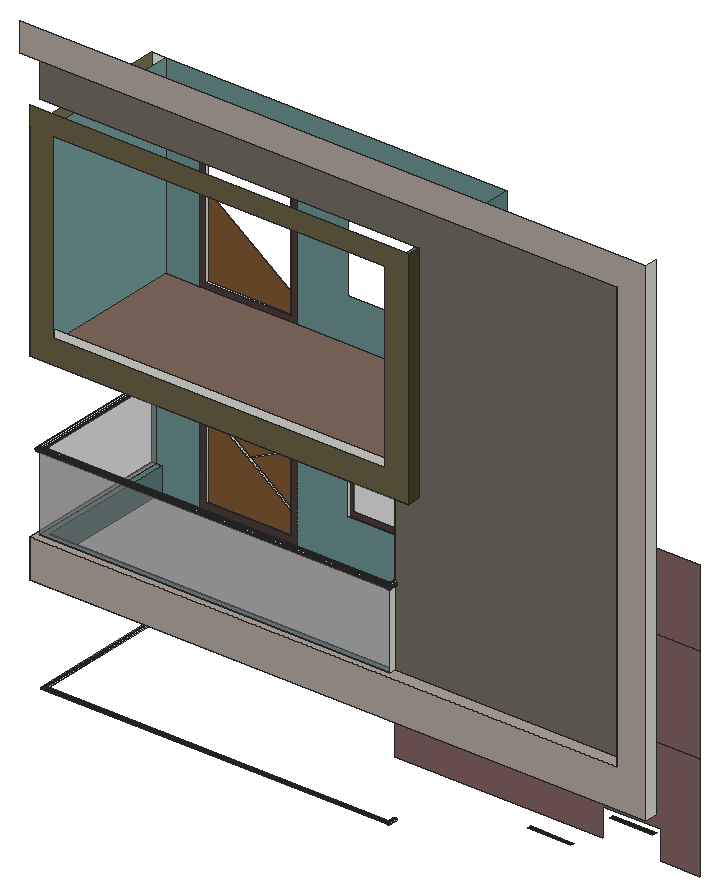
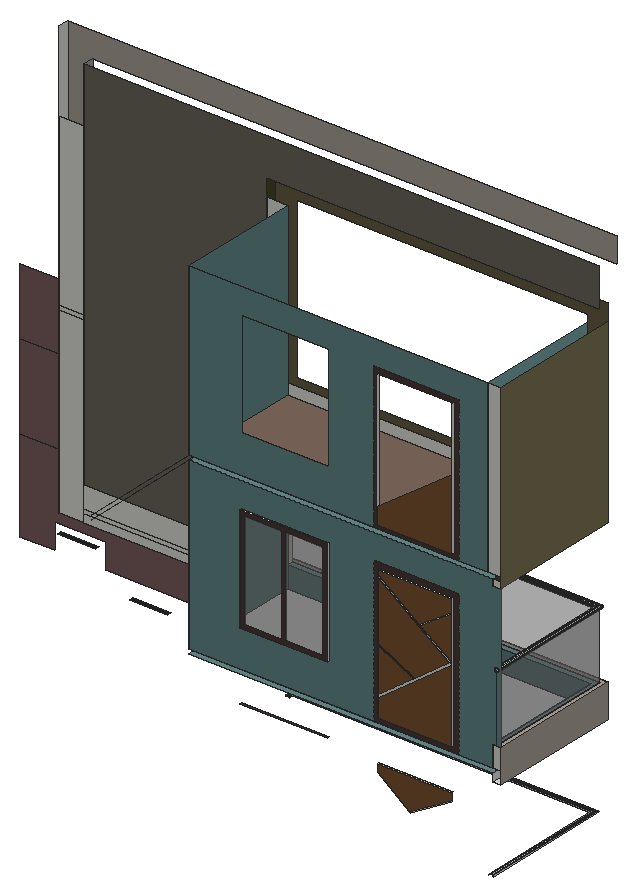
# SketchUp Ruby script. Lengths in inches.
U = 1.inch
M = Sketchup.active_model
def pt(a) = Geom::Point3d.new(a.map { |v| v * U })
def face(e, loops, mat)
  f = e.add_face(loops[0].map { |a| pt(a) })
  loops[1..].each { |l| e.add_face(l.map { |a| pt(a) }).erase! }
  f.material = f.back_material = mat if mat
  f
end
# faces: each face lists its corners as indices into pts; further lists are holes
def faces(e, pts, list, mat = nil) = list.each { |f| face(e, (f[0].is_a?(Array) ? f : [f]).map { |l| l.map { |i| pts[i] } }, mat) }
# xy, xz, yz: faces in a plane at the given z, y or x. An outline is a flat list of corners, or four numbers for a rectangle; further outlines are holes
def ring(l) = l.size == 4 ? [[l[0], l[1]], [l[2], l[1]], [l[2], l[3]], [l[0], l[3]]] : l.each_slice(2).to_a
def flat(e, list, mat, &to3) = list.each { |f| face(e, (f[0].is_a?(Array) ? f : [f]).map { |l| ring(l).map { |u, v| to3.(u, v) } }, mat) }
def xy(e, z, list, mat = nil) = flat(e, list, mat) { |x, y| [x, y, z] }
def xz(e, y, list, mat = nil) = flat(e, list, mat) { |x, z| [x, y, z] }
def yz(e, x, list, mat = nil) = flat(e, list, mat) { |y, z| [x, y, z] }
def lines(e, pts, list) = list.each { |a, b| e.add_line(pt(pts[a]), pt(pts[b])) }
# prism: a flat outline (further loops are holes) pulled along v
def prism(e, loops, v, mat = nil)
  f = face(e, loops, mat); d = Geom::Vector3d.new(v.map { |x| x * U })
  f.pushpull(f.normal.samedirection?(d) ? d.length : -d.length)
end
def box(e, o, s, mat = nil) = prism(e, [[o, [o[0] + s[0], o[1], o[2]], [o[0] + s[0], o[1] + s[1], o[2]], [o[0], o[1] + s[1], o[2]]]], [0, 0, s[2]], mat)
def at(x, y, z, deg = 0) = Geom::Transformation.translation(pt([x, y, z])) * Geom::Transformation.rotation(ORIGIN, Z_AXIS, deg.degrees)
def axes(o, x, y, z) = Geom::Transformation.new([*x, 0, *y, 0, *z, 0, *pt(o).to_a, 1])
def part(name) = M.definitions.add(name)
# library, detail: a bought-in or finely detailed component or shape, given as its bounding box
def library(name, o, s) = part(name).tap { |d| box(d.entities, o, s) }
def detail(e, o, s) = box(e.add_group.entities, o, s)
def put(e, d, t, mat = nil) = e.add_instance(d, t).tap { |i| i.material = mat if mat }
def group(e, t, mat = nil) = e.add_group.tap { |g| g.transformation = t; g.material = mat if mat }.entities
root = M.entities
M.materials.add("[0057_DarkKhaki]").color = [71, 69, 40]
M.materials.add("[0089_PaleTurquoise]").color = [103, 140, 140]
M.materials.add("[0089_PaleTurquoise]1").color = [120, 163, 163]
M.materials.add("[0089_PaleTurquoise]2").color = [93, 127, 127]
M.materials.add("[0119_RosyBrown]").color = [127, 96, 96]
M.materials.add("[0119_RosyBrown]1").color = [76, 58, 58]
M.materials.add("[0136_Charcoal]").color = [35, 35, 35]
M.materials.add("[Carrera Marble]").color = [193, 193, 193]
M.materials.add("[Cladding Stucco White]").color = [173, 163, 155]
M.materials.add("[Cladding Weathered]").color = [111, 105, 96]
M.materials.add("[Granite Brown]").color = [126, 104, 91]
M.materials.add("[Translucent Glass Gray]").color = [130, 130, 130]
M.materials["[Translucent Glass Gray]"].alpha = 0.5
M.materials.add("[Translucent Glass Gray]1").color = [128, 128, 128]
M.materials["[Translucent Glass Gray]1"].alpha = 0.5
M.materials.add("[Wood Floor]").color = [124, 84, 49]
M.materials.add("[Wood Lumber ButtJoined]").color = [102, 94, 69]
M.materials.add("[Wood Lumber ButtJoined]1").color = [127, 118, 87]
xy(root,1310.4375,[[1452,198,1560,208]],"[0136_Charcoal]")
xy(root,1388.4,[[375.6,546,584.4,551]])
xy(root,1404,[[726,546,973.25,552]],"[0119_RosyBrown]1")
xy(root,1406.375,[[1656,198,1764,208]],"[0136_Charcoal]")
xy(root,1452,[[240,167,240,546,264,546,264,198,1770,198,1770,167]])
xy(root,1476,[[353.9,283.84,350.8,284.25,347.9,285.44,345.42,287.35,343.51,289.84,342.31,292.73,341.9,295.84,342.31,298.94,343.51,301.84,345.42,304.32,347.9,306.23,350.8,307.43,353.9,307.84,357.01,307.43,359.9,306.23,362.39,304.32,364.29,301.84,365.49,298.94,365.9,295.84,365.49,292.73,364.29,289.84,362.39,287.35,359.9,285.44,357.01,284.25],[677.9,283.84,674.8,284.25,671.9,285.44,669.42,287.35,667.51,289.84,666.31,292.73,665.9,295.84,666.31,298.94,667.51,301.84,669.42,304.32,671.9,306.23,674.8,307.43,677.9,307.84,681.01,307.43,683.9,306.23,686.39,304.32,688.29,301.84,689.49,298.94,689.9,295.84,689.49,292.73,688.29,289.84,686.39,287.35,683.9,285.44,681.01,284.25],[1001.9,283.84,998.8,284.25,995.9,285.44,993.42,287.35,991.51,289.84,990.31,292.73,989.9,295.84,990.31,298.94,991.51,301.84,993.42,304.32,995.9,306.23,998.8,307.43,1001.9,307.84,1005.01,307.43,1007.9,306.23,1010.39,304.32,1012.29,301.84,1013.49,298.94,1013.9,295.84,1013.49,292.73,1012.29,289.84,1010.39,287.35,1007.9,285.44,1005.01,284.25],[353.9,403.84,350.8,404.25,347.9,405.44,345.42,407.35,343.51,409.84,342.31,412.73,341.9,415.84,342.31,418.94,343.51,421.84,345.42,424.32,347.9,426.23,350.8,427.43,353.9,427.84,357.01,427.43,359.9,426.23,362.39,424.32,364.29,421.84,365.49,418.94,365.9,415.84,365.49,412.73,364.29,409.84,362.39,407.35,359.9,405.44,357.01,404.25],[677.9,403.84,674.8,404.25,671.9,405.44,669.42,407.35,667.51,409.84,666.31,412.73,665.9,415.84,666.31,418.94,667.51,421.84,669.42,424.32,671.9,426.23,674.8,427.43,677.9,427.84,681.01,427.43,683.9,426.23,686.39,424.32,688.29,421.84,689.49,418.94,689.9,415.84,689.49,412.73,688.29,409.84,686.39,407.35,683.9,405.44,681.01,404.25],
  [1001.9,403.84,998.8,404.25,995.9,405.44,993.42,407.35,991.51,409.84,990.31,412.73,989.9,415.84,990.31,418.94,991.51,421.84,993.42,424.32,995.9,426.23,998.8,427.43,1001.9,427.84,1005.01,427.43,1007.9,426.23,1010.39,424.32,1012.29,421.84,1013.49,418.94,1013.9,415.84,1013.49,412.73,1012.29,409.84,1010.39,407.35,1007.9,405.44,1005.01,404.25]])
xy(root,1476,[[[264,198,1122,546],[353.9,403.84,357.01,404.25,359.9,405.44,362.39,407.35,364.29,409.84,365.49,412.73,365.9,415.84,365.49,418.94,364.29,421.84,362.39,424.32,359.9,426.23,357.01,427.43,353.9,427.84,350.8,427.43,347.9,426.23,345.42,424.32,343.51,421.84,342.31,418.94,341.9,415.84,342.31,412.73,343.51,409.84,345.42,407.35,347.9,405.44,350.8,404.25],[353.9,283.84,357.01,284.25,359.9,285.44,362.39,287.35,364.29,289.84,365.49,292.73,365.9,295.84,365.49,298.94,364.29,301.84,362.39,304.32,359.9,306.23,357.01,307.43,353.9,307.84,350.8,307.43,347.9,306.23,345.42,304.32,343.51,301.84,342.31,298.94,341.9,295.84,342.31,292.73,343.51,289.84,345.42,287.35,347.9,285.44,350.8,284.25],[677.9,403.84,681.01,404.25,683.9,405.44,686.39,407.35,688.29,409.84,689.49,412.73,689.9,415.84,689.49,418.94,688.29,421.84,686.39,424.32,683.9,426.23,681.01,427.43,677.9,427.84,674.8,427.43,671.9,426.23,669.42,424.32,667.51,421.84,666.31,418.94,665.9,415.84,666.31,412.73,667.51,409.84,669.42,407.35,671.9,405.44,674.8,404.25],[677.9,283.84,681.01,284.25,683.9,285.44,686.39,287.35,688.29,289.84,689.49,292.73,689.9,295.84,689.49,298.94,688.29,301.84,686.39,304.32,683.9,306.23,681.01,307.43,677.9,307.84,674.8,307.43,671.9,306.23,669.42,304.32,667.51,301.84,666.31,298.94,665.9,295.84,666.31,292.73,667.51,289.84,669.42,287.35,671.9,285.44,674.8,284.25],[1001.9,283.84,1005.01,284.25,1007.9,285.44,1010.39,287.35,1012.29,289.84,1013.49,292.73,1013.9,295.84,1013.49,298.94,1012.29,301.84,1010.39,304.32,1007.9,306.23,1005.01,307.43,1001.9,307.84,998.8,307.43,995.9,306.23,993.42,304.32,991.51,301.84,990.31,298.94,989.9,295.84,990.31,292.73,991.51,289.84,993.42,287.35,995.9,285.44,998.8,284.25],[1001.9,403.84,1005.01,404.25,1007.9,405.44,1010.39,407.35,1012.29,409.84,1013.49,412.73,1013.9,415.84,1013.49,418.94,1012.29,421.84,1010.39,424.32,1007.9,426.23,1005.01,427.43,1001.9,427.84,998.8,427.43,995.9,426.23,993.42,424.32,991.51,421.84,990.31,418.94,989.9,415.84,990.31,412.73,991.51,409.84,993.42,407.35,995.9,405.44,998.8,404.25]]],"[0089_PaleTurquoise]")
xy(root,1488,[[264,198,1122,546]],"[Carrera Marble]")
xy(root,1503.6,[[375.6,546,584.4,551]])
xy(root,1548,[[252,182.5,1122,182.5,1122,198,264,198,264,546,252,546]],"[0089_PaleTurquoise]2")
xy(root,1548,[[240,167,1698,167,1698,198,1122,198,1122,182.5,252,182.5,252,546,240,546]],"[Cladding Stucco White]")
xy(root,1596,[[726,546,973.25,552]])
xy(root,1880.4,[[375.6,546,584.4,551]])
xy(root,1896,[[726,546,973.25,552]])
xy(root,1950,[[240,167,240,546,264,546,264,191,1122,191,1122,198,1182,198,1182,167]],"[0057_DarkKhaki]")
xy(root,1968,[[353.9,283.84,350.8,284.25,347.9,285.44,345.42,287.35,343.51,289.84,342.31,292.73,341.9,295.84,342.31,298.94,343.51,301.84,345.42,304.32,347.9,306.23,350.8,307.43,353.9,307.84,357.01,307.43,359.9,306.23,362.39,304.32,364.29,301.84,365.49,298.94,365.9,295.84,365.49,292.73,364.29,289.84,362.39,287.35,359.9,285.44,357.01,284.25],[677.9,283.84,674.8,284.25,671.9,285.44,669.42,287.35,667.51,289.84,666.31,292.73,665.9,295.84,666.31,298.94,667.51,301.84,669.42,304.32,671.9,306.23,674.8,307.43,677.9,307.84,681.01,307.43,683.9,306.23,686.39,304.32,688.29,301.84,689.49,298.94,689.9,295.84,689.49,292.73,688.29,289.84,686.39,287.35,683.9,285.44,681.01,284.25],[1001.9,283.84,998.8,284.25,995.9,285.44,993.42,287.35,991.51,289.84,990.31,292.73,989.9,295.84,990.31,298.94,991.51,301.84,993.42,304.32,995.9,306.23,998.8,307.43,1001.9,307.84,1005.01,307.43,1007.9,306.23,1010.39,304.32,1012.29,301.84,1013.49,298.94,1013.9,295.84,1013.49,292.73,1012.29,289.84,1010.39,287.35,1007.9,285.44,1005.01,284.25],[353.9,403.84,350.8,404.25,347.9,405.44,345.42,407.35,343.51,409.84,342.31,412.73,341.9,415.84,342.31,418.94,343.51,421.84,345.42,424.32,347.9,426.23,350.8,427.43,353.9,427.84,357.01,427.43,359.9,426.23,362.39,424.32,364.29,421.84,365.49,418.94,365.9,415.84,365.49,412.73,364.29,409.84,362.39,407.35,359.9,405.44,357.01,404.25],[677.9,403.84,674.8,404.25,671.9,405.44,669.42,407.35,667.51,409.84,666.31,412.73,665.9,415.84,666.31,418.94,667.51,421.84,669.42,424.32,671.9,426.23,674.8,427.43,677.9,427.84,681.01,427.43,683.9,426.23,686.39,424.32,688.29,421.84,689.49,418.94,689.9,415.84,689.49,412.73,688.29,409.84,686.39,407.35,683.9,405.44,681.01,404.25],
  [1001.9,403.84,998.8,404.25,995.9,405.44,993.42,407.35,991.51,409.84,990.31,412.73,989.9,415.84,990.31,418.94,991.51,421.84,993.42,424.32,995.9,426.23,998.8,427.43,1001.9,427.84,1005.01,427.43,1007.9,426.23,1010.39,424.32,1012.29,421.84,1013.49,418.94,1013.9,415.84,1013.49,412.73,1012.29,409.84,1010.39,407.35,1007.9,405.44,1005.01,404.25]])
xy(root,1968,[[[264,191,1122,546],[1001.9,283.84,1005.01,284.25,1007.9,285.44,1010.39,287.35,1012.29,289.84,1013.49,292.73,1013.9,295.84,1013.49,298.94,1012.29,301.84,1010.39,304.32,1007.9,306.23,1005.01,307.43,1001.9,307.84,998.8,307.43,995.9,306.23,993.42,304.32,991.51,301.84,990.31,298.94,989.9,295.84,990.31,292.73,991.51,289.84,993.42,287.35,995.9,285.44,998.8,284.25],[1001.9,403.84,1005.01,404.25,1007.9,405.44,1010.39,407.35,1012.29,409.84,1013.49,412.73,1013.9,415.84,1013.49,418.94,1012.29,421.84,1010.39,424.32,1007.9,426.23,1005.01,427.43,1001.9,427.84,998.8,427.43,995.9,426.23,993.42,424.32,991.51,421.84,990.31,418.94,989.9,415.84,990.31,412.73,991.51,409.84,993.42,407.35,995.9,405.44,998.8,404.25],[353.9,283.84,357.01,284.25,359.9,285.44,362.39,287.35,364.29,289.84,365.49,292.73,365.9,295.84,365.49,298.94,364.29,301.84,362.39,304.32,359.9,306.23,357.01,307.43,353.9,307.84,350.8,307.43,347.9,306.23,345.42,304.32,343.51,301.84,342.31,298.94,341.9,295.84,342.31,292.73,343.51,289.84,345.42,287.35,347.9,285.44,350.8,284.25],[353.9,403.84,357.01,404.25,359.9,405.44,362.39,407.35,364.29,409.84,365.49,412.73,365.9,415.84,365.49,418.94,364.29,421.84,362.39,424.32,359.9,426.23,357.01,427.43,353.9,427.84,350.8,427.43,347.9,426.23,345.42,424.32,343.51,421.84,342.31,418.94,341.9,415.84,342.31,412.73,343.51,409.84,345.42,407.35,347.9,405.44,350.8,404.25],[677.9,283.84,681.01,284.25,683.9,285.44,686.39,287.35,688.29,289.84,689.49,292.73,689.9,295.84,689.49,298.94,688.29,301.84,686.39,304.32,683.9,306.23,681.01,307.43,677.9,307.84,674.8,307.43,671.9,306.23,669.42,304.32,667.51,301.84,666.31,298.94,665.9,295.84,666.31,292.73,667.51,289.84,669.42,287.35,671.9,285.44,674.8,284.25],[677.9,403.84,681.01,404.25,683.9,405.44,686.39,407.35,688.29,409.84,689.49,412.73,689.9,415.84,689.49,418.94,688.29,421.84,686.39,424.32,683.9,426.23,681.01,427.43,677.9,427.84,674.8,427.43,671.9,426.23,669.42,424.32,667.51,421.84,666.31,418.94,665.9,415.84,666.31,412.73,667.51,409.84,669.42,407.35,671.9,405.44,674.8,404.25]]],"[0089_PaleTurquoise]")
xy(root,1980,[[276,198,1122,546]],"[Granite Brown]")
xy(root,1993.89,[[373.89,546,586.11,552]])
xz(root,167,[[240,1452,1770,1452,1770,2688,216,2688,216,2616,1698,2616,1698,1548,240,1548]],"[Cladding Stucco White]")
xz(root,167,[[[240,1950,1182,2508],[296.4,2010,1122,2460]]],"[Wood Lumber ButtJoined]")
xz(root,182.5,[[252,1548,1122,1734]],"[Translucent Glass Gray]")
xz(root,191,[[264,1950,1122,1968]],"[0057_DarkKhaki]")
xz(root,198,[[264,1452,1122,1476],[1122,1452,1698,1476],[1698,1452,1770,1968],[1122,1476,1698,1488],[1122,1488,1698,1548],
  [1122,1968,1182,1980],[1698,1968,1770,1980],[276,1980,1122,2010],[1122,1980,1182,2460],[1698,1980,1770,2460]])
xz(root,198,[[264,1488,1122,1548]],"[0089_PaleTurquoise]2")
xz(root,198,[[1122,1353.5,1638,1353.5,1638,1424.375,1782,1424.375,1782,1353.5,1879.2,1353.5,1879.2,1614.875,1770,1614.875,1770,1452,1122,1452],[1770,1614.875,1879.2,1854.875],[1770,1854.875,1879.2,2046.875]],"[0119_RosyBrown]")
xz(root,198,[[1122,1548,1698,1548,1698,2616,240,2616,240,2508,1182,2508,1182,1950,1122,1950,1122,1746,1123.55,1745.8,1125,1745.2,1126.24,1744.24,1127.2,1743,1127.8,1741.55,1128,1740,1127.8,1738.45,1127.2,1737,1126.24,1735.76,1125,1734.8,1123.55,1734.2,1122,1734]],"[Cladding Weathered]")
xz(root,546,[[240,1488,264,1548],[252,1734,250.45,1734.2,249,1734.8,247.76,1735.76,246.8,1737,246.2,1738.45,246,1740,246.2,1741.55,246.8,1743,247.76,1744.24,249,1745.2,250.45,1745.8,252,1746,253.55,1745.8,255,1745.2,256.24,1744.24,257.2,1743,257.8,1741.55,258,1740,257.8,1738.45,257.2,1737,256.24,1735.76,255,1734.8,253.55,1734.2],[240,1950,264,1968],[240,1980,276,2460]])
xz(root,546,[[[264,1488,360,1488,360,1896,600,1896,600,1488,1122,1488,1122,1968,264,1968,264,1950,240,1950,240,1548,252,1548,252,1734,250.45,1734.2,249,1734.8,247.76,1735.76,246.8,1737,246.2,1738.45,246,1740,246.2,1741.55,246.8,1743,247.76,1744.24,249,1745.2,250.45,1745.8,252,1746,253.55,1745.8,255,1745.2,256.24,1744.24,257.2,1743,257.8,1741.55,258,1740,257.8,1738.45,257.2,1737,256.24,1735.76,255,1734.8,253.55,1734.2,252,1734,252,1548,264,1548],[726,1596,973.25,1896]],[[276,1980,360,1980,360,2388,600,2388,600,1980,1122,1980,1122,2460,276,2460],[726,2088,973.25,2388]]],"[0089_PaleTurquoise]")
xz(root,546,[[[360,1488,600,1896],[375.6,1503.6,584.4,1880.4]],[[360,1980,600,2388],[373.89,1993.89,586.11,2374.11]]],"[0119_RosyBrown]1")
xz(root,551,[[490.26,1296.05,493.62,1298.62,375.6,1368.29,375.6,1364.68],[584.4,1554.79,584.4,1561.87,482.2,1638.17,478.94,1640.6,380,1714.48,375.6,1711.28],[482.2,1638.17,584.4,1689.41,584.4,1692.55,478.94,1640.6],[375.6,1711.28,380,1714.48,584.4,1863,584.4,1866.41,467.39,1782.24,464.93,1780.47,375.6,1716.21],[464.93,1780.47,467.39,1782.24,375.6,1843.14,375.6,1840.87]])
xz(root,551,[[493.62,1298.62,584.4,1368.29,584.4,1388.4,375.6,1388.4,375.6,1368.29],[375.6,1503.6,584.4,1503.6,584.4,1554.79,375.6,1711.28],[584.4,1561.87,584.4,1689.41,482.2,1638.17],[478.94,1640.6,584.4,1692.55,584.4,1863,380,1714.48],[375.6,1716.21,464.93,1780.47,375.6,1840.87],
  [467.39,1782.24,584.4,1866.41,584.4,1880.4,375.6,1880.4,375.6,1843.14]],"[Wood Floor]")
xz(root,552,[[[726,1596,973.25,1896],[855.625,1608,961.25,1884],[738,1608,843.625,1884]]],"[0119_RosyBrown]1")
xz(root,552,[[738,1608,843.625,1884],[855.625,1608,961.25,1884]],"[Translucent Glass Gray]1")
xz(root,552,[[373.89,1993.89,586.11,1993.89,586.11,2039.4,373.89,2194.56]],"[Wood Floor]")
yz(root,240,[[167,1452,546,1548]],"[Cladding Stucco White]")
yz(root,240,[[167,1950,546,2460]],"[Wood Lumber ButtJoined]1")
yz(root,252,[[182.5,1548,546,1734]],"[Translucent Glass Gray]")
yz(root,264,[[198,1452,546,1476]])
yz(root,264,[[191,1950,546,1968]],"[0057_DarkKhaki]")
yz(root,264,[[198,1488,546,1548]],"[0089_PaleTurquoise]2")
yz(root,276,[[198,1980,546,2460]],"[0089_PaleTurquoise]1")
yz(root,373.89,[[546,1993.89,552,2374.11]])
yz(root,375.6,[[546,1503.6,551,1880.4]])
yz(root,584.4,[[546,1503.6,551,1880.4]])
yz(root,586.11,[[546,1993.89,552,2374.11]])
yz(root,726,[[546,1596,552,1896]])
yz(root,973.25,[[546,1596,552,1896]])
yz(root,1122,[[182.5,1548,198,1734],[182.5,1734,198,1740],[191,1950,198,1968]])
yz(root,1122,[[198,1488,546,1968],[198,1980,546,2460]],"[0089_PaleTurquoise]")
yz(root,1182,[[167,1950,198,2508]],"[0057_DarkKhaki]")
yz(root,1698,[[167,1548,198,2616]],"[Cladding Stucco White]")
yz(root,1770,[[167,1452,198,2688]])
p = [[261.8,174.8,1215],[261.2,174.2,1213.55],[1127.8,174.2,1213.55],[1127.2,174.8,1215],[261.8,546,1215],[261.2,546,1213.55],
  [1127.8,198,1213.55],[1127.2,198,1215],[272.8,185.8,1213.55],[272.2,185.2,1215],[1116.8,185.2,1215],[1116.2,185.8,1213.55],
  [272.8,546,1213.55],[272.2,546,1215],[1116.8,198,1215],[1116.2,198,1213.55],[262.76,175.76,1216.24],[1126.24,175.76,1216.24],
  [262.76,546,1216.24],[1126.24,198,1216.24],[271.24,184.24,1216.24],[1117.76,184.24,1216.24],[271.24,546,1216.24],[1117.76,198,1216.24],
  [264,177,1217.2],[1125,177,1217.2],[264,546,1217.2],[1125,198,1217.2],[270,183,1217.2],[1119,183,1217.2],
  [270,546,1217.2],[1119,198,1217.2],[265.45,178.45,1217.8],[1123.55,178.45,1217.8],[265.45,546,1217.8],[1123.55,198,1217.8],
  [268.55,181.55,1217.8],[1120.45,181.55,1217.8],[268.55,546,1217.8],[1120.45,198,1217.8],[267,180,1218],[1122,180,1218],
  [267,546,1218],[1122,198,1218],[250.45,546,1734.2],[252,546,1734],[252,182.5,1734],[250.45,180.95,1734.2],
  [1122,182.5,1734],[1123.55,180.95,1734.2],[1122,198,1734],[1123.55,198,1734.2],[253.55,546,1734.2],[253.55,184.05,1734.2],
  [1120.45,184.05,1734.2],[1120.45,198,1734.2],[249,546,1734.8],[249,179.5,1734.8],[1125,179.5,1734.8],[1125,198,1734.8],
  [255,546,1734.8],[255,185.5,1734.8],[1119,185.5,1734.8],[1119,198,1734.8],[247.76,546,1735.76],[247.76,178.26,1735.76],
  [1126.24,178.26,1735.76],[1126.24,198,1735.76],[256.24,546,1735.76],[256.24,186.74,1735.76],[1117.76,186.74,1735.76],[1117.76,198,1735.76],
  [246.8,546,1737],[246.8,177.3,1737],[1127.2,177.3,1737],[1127.2,198,1737],[257.2,546,1737],[257.2,187.7,1737],
  [1116.8,187.7,1737],[1116.8,198,1737],[246.2,546,1738.45],[246.2,176.7,1738.45],[1127.8,176.7,1738.45],[1127.8,198,1738.45],
  [257.8,546,1738.45],[257.8,188.3,1738.45],[1116.2,188.3,1738.45],[1116.2,198,1738.45],[246,546,1740],[246,176.5,1740],
  [1128,176.5,1740],[1128,198,1740],[258,546,1740],[258,188.5,1740],[1116,188.5,1740],[1116,198,1740],
  [246.2,546,1741.55],[246.2,176.7,1741.55],[1127.8,176.7,1741.55],[1127.8,198,1741.55],[257.8,546,1741.55],[257.8,188.3,1741.55],
  [1116.2,188.3,1741.55],[1116.2,198,1741.55],[246.8,546,1743],[246.8,177.3,1743],[1127.2,177.3,1743],[1127.2,198,1743],
  [257.2,546,1743],[257.2,187.7,1743],[1116.8,187.7,1743],[1116.8,198,1743],[247.76,546,1744.24],[247.76,178.26,1744.24],
  [1126.24,178.26,1744.24],[1126.24,198,1744.24],[256.24,546,1744.24],[256.24,186.74,1744.24],[1117.76,186.74,1744.24],[1117.76,198,1744.24],
  [249,546,1745.2],[249,179.5,1745.2],[1125,179.5,1745.2],[1125,198,1745.2],[255,546,1745.2],[255,185.5,1745.2],
  [1119,185.5,1745.2],[1119,198,1745.2],[250.45,546,1745.8],[250.45,180.95,1745.8],[1123.55,180.95,1745.8],[1123.55,198,1745.8],
  [253.55,546,1745.8],[253.55,184.05,1745.8],[1120.45,184.05,1745.8],[1120.45,198,1745.8],[252,546,1746],[252,182.5,1746],
  [1122,182.5,1746],[1122,198,1746],[1122,546,1968],[1122,894,1968],[1122,546,1980],[1122,894,1980],
  [252,182.5,1740],[252,546,1740],[1122,182.5,1740]]
faces(root,p,[[0,1,2,3],[4,5,1,0],[3,2,6,7],[8,9,10,11],[12,13,9,8],[11,10,14,15],[16,0,3,17],[18,4,0,16],
  [17,3,7,19],[9,20,21,10],[13,22,20,9],[10,21,23,14],[24,16,17,25],[26,18,16,24],[25,17,19,27],[20,28,29,21],
  [22,30,28,20],[21,29,31,23],[32,24,25,33],[34,26,24,32],[33,25,27,35],[28,36,37,29],[30,38,36,28],[29,37,39,31],
  [40,32,33,41],[42,34,32,40],[41,33,35,43],[36,40,41,37],[38,42,40,36],[37,41,43,39],[44,45,46,47],[47,46,48,49],
  [49,48,50,51],[45,52,53,46],[46,53,54,48],[48,54,55,50],[56,44,47,57],[57,47,49,58],[58,49,51,59],[52,60,61,53],
  [53,61,62,54],[54,62,63,55],[64,56,57,65],[65,57,58,66],[66,58,59,67],[60,68,69,61],[61,69,70,62],[62,70,71,63],
  [72,64,65,73],[73,65,66,74],[74,66,67,75],[68,76,77,69],[69,77,78,70],[70,78,79,71],[80,72,73,81],[81,73,74,82],
  [82,74,75,83],[76,84,85,77],[77,85,86,78],[78,86,87,79],[88,80,81,89],[89,81,82,90],[90,82,83,91],[84,92,93,85],
  [85,93,94,86],[86,94,95,87],[96,88,89,97],[97,89,90,98],[98,90,91,99],[92,100,101,93],[93,101,102,94],[94,102,103,95],
  [104,96,97,105],[105,97,98,106],[106,98,99,107],[100,108,109,101],[101,109,110,102],[102,110,111,103],[112,104,105,113],[113,105,106,114],
  [114,106,107,115],[108,116,117,109],[109,117,118,110],[110,118,119,111],[120,112,113,121],[121,113,114,122],[122,114,115,123],[116,124,125,117],
  [117,125,126,118],[118,126,127,119],[128,120,121,129],[129,121,122,130],[130,122,123,131],[124,132,133,125],[125,133,134,126],[126,134,135,127],
  [136,128,129,137],[137,129,130,138],[138,130,131,139],[132,136,137,133],[133,137,138,134],[134,138,139,135]])
lines(root,p,[[140,141],[142,143],[144,145],[144,146],[46,144]])
